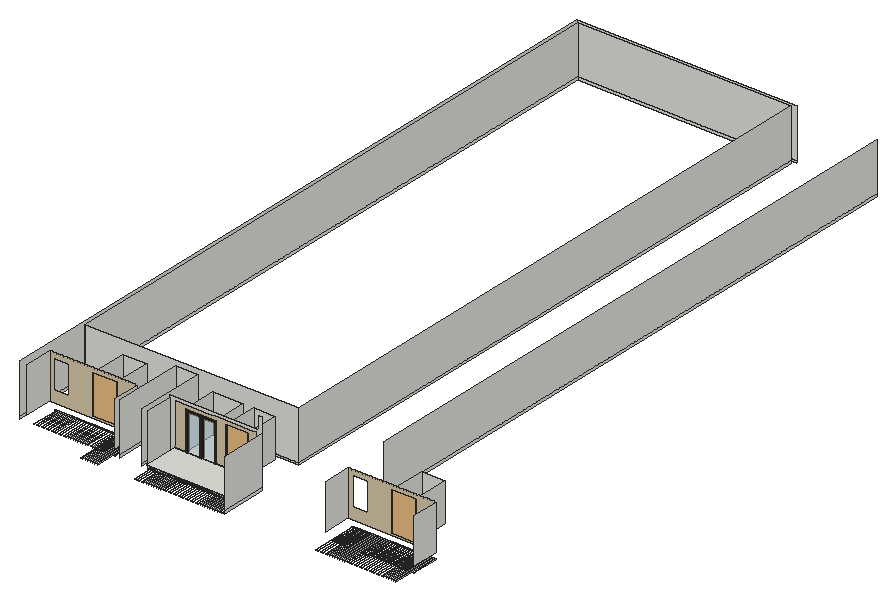
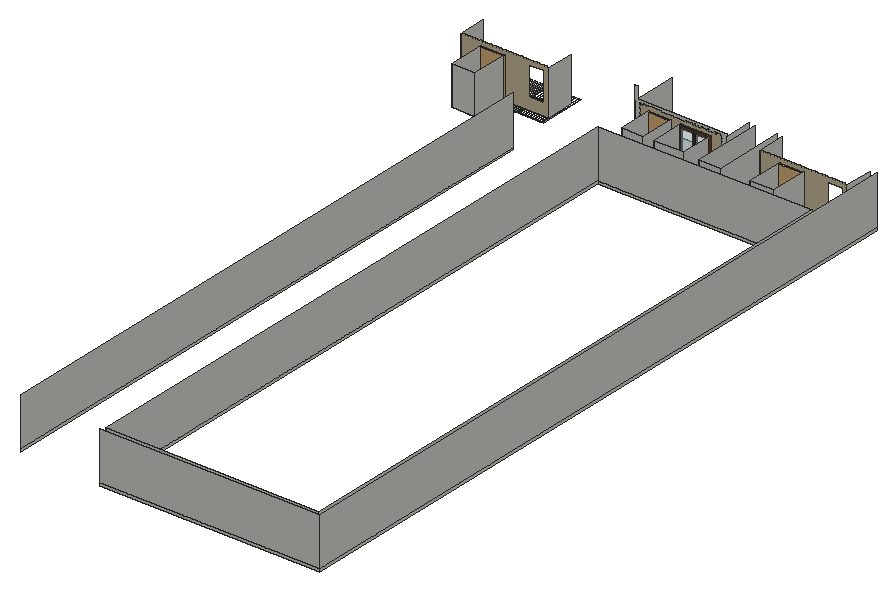
# SketchUp Ruby script. Lengths in inches.
U = 1.inch
M = Sketchup.active_model
def pt(a) = Geom::Point3d.new(a.map { |v| v * U })
def face(e, loops, mat)
  f = e.add_face(loops[0].map { |a| pt(a) })
  loops[1..].each { |l| e.add_face(l.map { |a| pt(a) }).erase! }
  f.material = f.back_material = mat if mat
  f
end
# faces: each face lists its corners as indices into pts; further lists are holes
def faces(e, pts, list, mat = nil) = list.each { |f| face(e, (f[0].is_a?(Array) ? f : [f]).map { |l| l.map { |i| pts[i] } }, mat) }
# xy, xz, yz: faces in a plane at the given z, y or x. An outline is a flat list of corners, or four numbers for a rectangle; further outlines are holes
def ring(l) = l.size == 4 ? [[l[0], l[1]], [l[2], l[1]], [l[2], l[3]], [l[0], l[3]]] : l.each_slice(2).to_a
def flat(e, list, mat, &to3) = list.each { |f| face(e, (f[0].is_a?(Array) ? f : [f]).map { |l| ring(l).map { |u, v| to3.(u, v) } }, mat) }
def xy(e, z, list, mat = nil) = flat(e, list, mat) { |x, y| [x, y, z] }
def xz(e, y, list, mat = nil) = flat(e, list, mat) { |x, z| [x, y, z] }
def yz(e, x, list, mat = nil) = flat(e, list, mat) { |y, z| [x, y, z] }
def lines(e, pts, list) = list.each { |a, b| e.add_line(pt(pts[a]), pt(pts[b])) }
# prism: a flat outline (further loops are holes) pulled along v
def prism(e, loops, v, mat = nil)
  f = face(e, loops, mat); d = Geom::Vector3d.new(v.map { |x| x * U })
  f.pushpull(f.normal.samedirection?(d) ? d.length : -d.length)
end
def box(e, o, s, mat = nil) = prism(e, [[o, [o[0] + s[0], o[1], o[2]], [o[0] + s[0], o[1] + s[1], o[2]], [o[0], o[1] + s[1], o[2]]]], [0, 0, s[2]], mat)
def at(x, y, z, deg = 0) = Geom::Transformation.translation(pt([x, y, z])) * Geom::Transformation.rotation(ORIGIN, Z_AXIS, deg.degrees)
def axes(o, x, y, z) = Geom::Transformation.new([*x, 0, *y, 0, *z, 0, *pt(o).to_a, 1])
def part(name) = M.definitions.add(name)
# library, detail: a bought-in or finely detailed component or shape, given as its bounding box
def library(name, o, s) = part(name).tap { |d| box(d.entities, o, s) }
def detail(e, o, s) = box(e.add_group.entities, o, s)
def put(e, d, t, mat = nil) = e.add_instance(d, t).tap { |i| i.material = mat if mat }
def group(e, t, mat = nil) = e.add_group.tap { |g| g.transformation = t; g.material = mat if mat }.entities
root = M.entities
M.materials.add("[Field Square Tile]").color = [216, 200, 168]
M.materials.add("[Translucent Glass Safety]").color = [204, 235, 244]
M.materials["[Translucent Glass Safety]"].alpha = 0.5
M.materials.add("[Wood Floor Parquet]").color = [140, 85, 37]
M.materials.add("[Wood Veneer 01]").color = [51, 28, 15]
M.materials.add("[Wood Veneer 01]1").color = [120, 70, 37]
c1 = library("元件\#5",[-4.39,0,0],[5.37,35.83,90.55])
c2 = part("Component\#1")
xy(c2.entities,0,[[0,0,6,48]],"[Wood Veneer 01]1")
xy(c2.entities,4,[[0,4,1.8125,44],[1.8125,4,6,44]])
xy(c2.entities,80,[[0,4,1.8125,44],[1.8125,4,6,44]])
xy(c2.entities,84,[[0,0,6,48]],"[Wood Veneer 01]1")
xz(c2.entities,0,[[0,0,6,84]],"[Wood Veneer 01]1")
xz(c2.entities,4,[[0,4,1.8125,80],[1.8125,4,6,80]])
xz(c2.entities,44,[[0,4,1.8125,80],[1.8125,4,6,80]])
xz(c2.entities,48,[[0,0,6,84]],"[Wood Veneer 01]1")
yz(c2.entities,0,[[[0,0,48,84],[4,4,44,80]]],"[Wood Veneer 01]1")
yz(c2.entities,1.8125,[[4,4,44,80]],"[Translucent Glass Safety]")
yz(c2.entities,6,[[[0,0,48,84],[4,4,44,80]]],"[Wood Veneer 01]")
c3 = part("Group\#3")
put(c3.entities,c2,at(0,0,0),"[Wood Veneer 01]")
g1 = group(c3.entities,at(0,48,0),"[Wood Veneer 01]")
xy(g1,0,[[0,0,6,48]],"[Wood Veneer 01]1")
xy(g1,4,[[0,4,1.8125,44],[1.8125,4,6,44]])
xy(g1,80,[[0,4,1.8125,44],[1.8125,4,6,44]])
xy(g1,84,[[0,0,6,48]],"[Wood Veneer 01]1")
xz(g1,0,[[0,0,6,84]],"[Wood Veneer 01]1")
xz(g1,4,[[0,4,1.8125,80],[1.8125,4,6,80]])
xz(g1,44,[[0,4,1.8125,80],[1.8125,4,6,80]])
xz(g1,48,[[0,0,6,84]],"[Wood Veneer 01]1")
yz(g1,0,[[[0,0,48,84],[4,4,44,80]]],"[Wood Veneer 01]1")
yz(g1,1.8125,[[4,4,44,80]],"[Translucent Glass Safety]")
yz(g1,6,[[[0,0,48,84],[4,4,44,80]]],"[Wood Veneer 01]")
xy(root,254.6875,[[614.76,246.64,616.96,361.27],[616.96,246.64,622,361.27]])
xy(root,274.4375,[[207.81,361.27,266.47,452.64],[941.37,361.27,1000.03,452.64]])
xy(root,275.125,[[409.32,273.33,609.07,361.27],[435.49,361.27,509.74,445.08],[534.92,361.27,587.67,445.08]])
xz(root,361.27,[[256.68,253.5625,261.43,254.6875],[262.68,253.5625,267.43,254.6875],[268.68,253.5625,273.43,254.6875],[274.68,253.5625,279.43,254.6875],[280.68,253.5625,285.43,254.6875],
  [286.68,253.5625,291.43,254.6875],[292.68,253.5625,297.43,254.6875],[298.68,253.5625,303.43,254.6875],[304.68,253.5625,309.43,254.6875],[310.68,253.5625,315.43,254.6875],
  [990.25,253.5625,995,254.6875],[996.25,253.5625,1001,254.6875],[1002.25,253.5625,1007,254.6875],[1008.25,253.5625,1013,254.6875],[1014.25,253.5625,1019,254.6875],
  [1020.25,253.5625,1025,254.6875],[1026.25,253.5625,1031,254.6875],[1032.25,253.5625,1037,254.6875],[1038.25,253.5625,1043,254.6875],[1044.25,253.5625,1049,254.6875],
  [244.68,253.875,249.43,254.625],[250.68,253.875,255.43,254.6875],[978.25,253.875,983,254.625],[984.25,253.875,989,254.6875],[112.68,253.9375,117.43,254.6875],
  [118.68,253.9375,123.43,254.6875],[124.68,253.9375,129.43,254.6875],[130.68,253.9375,135.43,254.6875],[136.68,253.9375,141.43,254.6875],[142.68,253.9375,147.43,254.6875],
  [148.68,253.9375,153.43,254.6875],[154.68,253.9375,159.43,254.6875],[160.68,253.9375,165.43,254.6875],[166.68,253.9375,171.43,254.6875],[172.68,253.9375,177.43,254.6875],
  [178.68,253.9375,183.43,254.6875],[184.68,253.9375,189.43,254.6875],[190.68,253.9375,195.43,254.6875],[196.68,253.9375,201.43,254.6875],[202.68,253.9375,207.43,254.6875],
  [208.68,253.9375,213.43,254.6875],[214.68,253.9375,219.43,254.6875],[220.68,253.9375,225.43,254.6875],[226.68,253.9375,231.43,254.6875],[232.68,253.9375,237.43,254.6875],
  [238.68,253.9375,243.43,254.6875],[396.57,253.9375,400.96,254.6875],[402.57,253.9375,406.96,254.6875],[408.57,253.9375,412.96,254.6875],[414.57,253.9375,418.96,254.6875],
  [420.57,253.9375,424.96,254.6875],[426.57,253.9375,430.96,254.6875],[432.57,253.9375,436.96,254.6875],[438.57,253.9375,442.96,254.6875],[444.57,253.9375,448.96,254.6875],
  [450.57,253.9375,454.96,254.6875],[456.57,253.9375,460.96,254.6875],[462.57,253.9375,466.96,254.6875],[468.57,253.9375,472.96,254.6875],[474.57,253.9375,478.96,254.6875],
  [480.57,253.9375,484.96,254.6875],[486.57,253.9375,490.96,254.6875],[492.57,253.9375,496.96,254.6875],[498.57,253.9375,502.96,254.6875],[504.57,253.9375,508.96,254.6875],
  [510.57,253.9375,514.96,254.6875],[516.57,253.9375,520.96,254.6875],[522.57,253.9375,526.96,254.6875],[528.57,253.9375,532.96,254.6875],[534.57,253.9375,538.96,254.6875],
  [540.57,253.9375,544.96,254.6875],[546.57,253.9375,550.96,254.6875],[552.57,253.9375,556.96,254.6875],[558.57,253.9375,562.96,254.6875],[564.57,253.9375,568.96,254.6875],
  [570.57,253.9375,574.96,254.6875],[576.57,253.9375,580.96,254.6875],[582.57,253.9375,586.96,254.6875],[588.57,253.9375,592.96,254.6875],[594.57,253.9375,598.96,254.6875],
  [600.57,253.9375,604.96,254.6875],[606.57,253.9375,610.96,254.6875],[612.57,253.9375,614.76,254.6875],[846.25,253.9375,851,254.6875],[852.25,253.9375,857,254.6875],
  [858.25,253.9375,863,254.6875],[864.25,253.9375,869,254.6875],[870.25,253.9375,875,254.6875],[876.25,253.9375,881,254.6875],[882.25,253.9375,887,254.6875],
  [888.25,253.9375,893,254.6875],[894.25,253.9375,899,254.6875],[900.25,253.9375,905,254.6875],[906.25,253.9375,911,254.6875],[912.25,253.9375,917,254.6875],
  [918.25,253.9375,923,254.6875],[924.25,253.9375,929,254.6875],[930.25,253.9375,935,254.6875],[936.25,253.9375,941,254.6875],[942.25,253.9375,947,254.6875],
  [948.25,253.9375,953,254.6875],[954.25,253.9375,959,254.6875],[960.25,253.9375,965,254.6875],[966.25,253.9375,971,254.6875],[972.25,253.9375,977,254.6875],
  [244.68,254.625,249.43,254.6875],[978.25,254.625,983,254.6875],[[396.57,254.6875,396.57,386.6875,614.76,386.6875,614.76,416.75,622,416.75,622,254.6875],[435.49,260.6875,509.74,260.6875,509.74,275.125,534.92,275.125,534.92,260.6875,587.67,260.6875,587.67,275.125,609.07,275.125,609.07,380.6875,605.74,380.6875,605.74,380.1875,601.32,380.1875,601.32,380.6875,599.74,380.6875,599.74,380.1875,595.32,380.1875,595.32,380.6875,593.74,380.6875,593.74,380.1875,589.32,380.1875,589.32,380.6875,587.74,380.6875,587.74,380.1875,583.32,380.1875,583.32,380.6875,581.74,380.6875,581.74,380.1875,577.32,380.1875,577.32,380.6875,575.74,380.6875,575.74,380.1875,571.32,380.1875,571.32,380.6875,569.74,380.6875,569.74,380.0625,565.32,380.0625,565.32,380.6875,563.74,380.6875,563.74,380.0625,559.32,380.0625,559.32,380.6875,557.74,380.6875,557.74,380.0625,553.32,380.0625,553.32,380.6875,551.74,380.6875,551.74,380.0625,547.32,380.0625,547.32,380.6875,545.74,380.6875,545.74,380.0625,541.32,380.0625,541.32,380.6875,539.74,380.6875,539.74,380.0625,535.32,380.0625,535.32,380.6875,533.74,380.6875,533.74,380.0625,529.32,380.0625,529.32,380.6875,527.74,380.6875,527.74,380.0625,523.32,380.0625,523.32,380.6875,521.74,380.6875,521.74,380.0625,517.32,380.0625,517.32,380.6875,515.74,380.6875,515.74,380.0625,511.32,380.0625,511.32,380.6875,509.74,380.6875,509.74,380.0625,505.32,380.0625,505.32,380.6875,503.74,380.6875,503.74,379.5625,499.32,379.5625,499.32,380.6875,497.74,380.6875,497.74,379.5625,493.32,379.5625,493.32,380.6875,491.74,380.6875,491.74,379.5625,487.32,379.5625,487.32,380.6875,485.74,380.6875,485.74,379.5625,481.32,379.5625,481.32,380.6875,479.74,380.6875,479.74,379.5625,475.32,379.5625,475.32,380.6875,473.74,380.6875,473.74,379.5625,469.32,379.5625,469.32,380.6875,467.74,380.6875,467.74,379.5625,463.32,379.5625,463.32,380.6875,461.74,380.6875,461.74,379.5625,457.32,379.5625,457.32,380.6875,455.74,380.6875,455.74,379.5625,451.32,379.5625,451.32,380.6875,449.74,380.6875,449.74,379.5625,445.32,379.5625,445.32,380.6875,443.74,380.6875,443.74,379.5625,439.32,379.5625,439.32,380.6875,437.74,380.6875,437.74,379.5625,433.32,379.5625,433.32,380.6875,431.74,380.6875,431.74,379.5625,427.32,379.5625,427.32,380.6875,425.74,380.6875,425.74,379.5625,421.32,379.5625,421.32,380.6875,419.74,380.6875,419.74,379.5625,415.32,379.5625,415.32,380.6875,413.74,380.6875,413.74,379.5625,409.32,379.5625,409.32,275.125,435.49,275.125]],[435.49,260.6875,509.74,275.125],[534.92,260.6875,587.67,275.125]])
xz(root,361.27,[[[100.18,269.0625,315.43,269.0625,315.43,378.875,310.4,378.875,310.4,380.6875,307.02,380.6875,307.02,378.875,301.98,378.875,301.98,380.6875,298.61,380.6875,298.61,378.875,293.57,378.875,293.57,380.6875,290.2,380.6875,290.2,378.875,285.16,378.875,285.16,380.6875,281.78,380.6875,281.78,378.875,276.75,378.875,276.75,380.6875,273.37,380.6875,273.37,378.875,268.33,378.875,268.33,380.6875,264.96,380.6875,264.96,378.875,259.92,378.875,259.92,380.6875,256.55,380.6875,256.55,378.875,251.51,378.875,251.51,380.6875,248.13,380.6875,248.13,378.875,243.1,378.875,243.1,380.6875,239.72,380.6875,239.72,378.875,234.68,378.875,234.68,380.6875,231.31,380.6875,231.31,378.875,226.27,378.875,226.27,380.6875,222.89,380.6875,222.89,378.875,217.86,378.875,217.86,380.6875,214.48,380.6875,214.48,378.875,209.44,378.875,209.44,380.6875,206.07,380.6875,206.07,378.875,201.03,378.875,201.03,380.6875,197.66,380.6875,197.66,378.875,192.62,378.875,192.62,380.6875,189.24,380.6875,189.24,378.875,184.21,378.875,184.21,380.6875,180.83,380.6875,180.83,378.875,175.79,378.875,175.79,380.6875,172.42,380.6875,172.42,378.875,167.38,378.875,167.38,380.6875,164.01,380.6875,164.01,378.875,158.97,378.875,158.97,380.6875,155.59,380.6875,155.59,378.875,150.55,378.875,150.55,380.6875,147.18,380.6875,147.18,378.875,142.14,378.875,142.14,380.6875,138.77,380.6875,138.77,378.875,133.73,378.875,133.73,380.6875,130.35,380.6875,130.35,378.875,125.32,378.875,125.32,380.6875,121.94,380.6875,121.94,378.875,116.9,378.875,116.9,380.6875,113.53,380.6875,113.53,378.875,108.49,378.875,108.49,380.6875,105.12,380.6875,105.12,378.875,100.18,378.875],[207.81,274.4375,266.47,369.36],[111.92,297.24,149.24,369.37]],[[833.74,269.0625,1049,269.0625,1049,378.875,1043.96,378.875,1043.96,380.6875,1040.58,380.6875,1040.58,378.875,1035.55,378.875,1035.55,380.6875,1032.17,380.6875,1032.17,378.875,1027.13,378.875,1027.13,380.6875,1023.76,380.6875,1023.76,378.875,1018.72,378.875,1018.72,380.6875,1015.35,380.6875,1015.35,378.875,1010.31,378.875,1010.31,380.6875,1006.93,380.6875,1006.93,378.875,1001.9,378.875,1001.9,380.6875,998.52,380.6875,998.52,378.875,993.48,378.875,993.48,380.6875,990.11,380.6875,990.11,378.875,985.07,378.875,985.07,380.6875,981.7,380.6875,981.7,378.875,976.66,378.875,976.66,380.6875,973.28,380.6875,973.28,378.875,968.24,378.875,968.24,380.6875,964.87,380.6875,964.87,378.875,959.83,378.875,959.83,380.6875,956.46,380.6875,956.46,378.875,951.42,378.875,951.42,380.6875,948.04,380.6875,948.04,378.875,943.01,378.875,943.01,380.6875,939.63,380.6875,939.63,378.875,934.59,378.875,934.59,380.6875,931.22,380.6875,931.22,378.875,926.18,378.875,926.18,380.6875,922.81,380.6875,922.81,378.875,917.77,378.875,917.77,380.6875,914.39,380.6875,914.39,378.875,909.36,378.875,909.36,380.6875,905.98,380.6875,905.98,378.875,900.94,378.875,900.94,380.6875,897.57,380.6875,897.57,378.875,892.53,378.875,892.53,380.6875,889.16,380.6875,889.16,378.875,884.12,378.875,884.12,380.6875,880.74,380.6875,880.74,378.875,875.7,378.875,875.7,380.6875,872.33,380.6875,872.33,378.875,867.29,378.875,867.29,380.6875,863.92,380.6875,863.92,378.875,858.88,378.875,858.88,380.6875,855.5,380.6875,855.5,378.875,850.47,378.875,850.47,380.6875,847.09,380.6875,847.09,378.875,842.05,378.875,842.05,380.6875,838.68,380.6875,838.68,378.875,833.74,378.875],[941.37,274.4375,1000.03,369.36],[845.49,297.24,882.8,369.37]],[409.32,275.125,435.49,275.125,435.49,369.625,509.74,369.625,509.74,275.125,534.92,275.125,534.92,369.6875,587.67,369.6875,587.67,275.125,609.07,275.125,609.07,380.6875,605.74,380.6875,605.74,380.1875,601.32,380.1875,601.32,380.6875,599.74,380.6875,599.74,380.1875,595.32,380.1875,595.32,380.6875,593.74,380.6875,593.74,380.1875,589.32,380.1875,589.32,380.6875,587.74,380.6875,587.74,380.1875,583.32,380.1875,583.32,380.6875,581.74,380.6875,581.74,380.1875,577.32,380.1875,577.32,380.6875,575.74,380.6875,575.74,380.1875,571.32,380.1875,571.32,380.6875,569.74,380.6875,569.74,380.0625,565.32,380.0625,565.32,380.6875,563.74,380.6875,563.74,380.0625,559.32,380.0625,559.32,380.6875,557.74,380.6875,557.74,380.0625,553.32,380.0625,553.32,380.6875,551.74,380.6875,551.74,380.0625,547.32,380.0625,547.32,380.6875,545.74,380.6875,545.74,380.0625,541.32,380.0625,541.32,380.6875,539.74,380.6875,539.74,380.0625,535.32,380.0625,535.32,380.6875,533.74,380.6875,533.74,380.0625,529.32,380.0625,529.32,380.6875,527.74,380.6875,527.74,380.0625,523.32,380.0625,523.32,380.6875,521.74,380.6875,521.74,380.0625,517.32,380.0625,517.32,380.6875,515.74,380.6875,515.74,380.0625,511.32,380.0625,511.32,380.6875,509.74,380.6875,509.74,380.0625,505.32,380.0625,505.32,380.6875,503.74,380.6875,503.74,379.5625,499.32,379.5625,499.32,380.6875,497.74,380.6875,497.74,379.5625,493.32,379.5625,493.32,380.6875,491.74,380.6875,491.74,379.5625,487.32,379.5625,487.32,380.6875,485.74,380.6875,485.74,379.5625,481.32,379.5625,481.32,380.6875,479.74,380.6875,479.74,379.5625,475.32,379.5625,475.32,380.6875,473.74,380.6875,473.74,379.5625,469.32,379.5625,469.32,380.6875,467.74,380.6875,467.74,379.5625,463.32,379.5625,463.32,380.6875,461.74,380.6875,461.74,379.5625,457.32,379.5625,457.32,380.6875,455.74,380.6875,455.74,379.5625,451.32,379.5625,451.32,380.6875,449.74,380.6875,449.74,379.5625,445.32,379.5625,445.32,380.6875,443.74,380.6875,443.74,379.5625,439.32,379.5625,439.32,380.6875,437.74,380.6875,437.74,379.5625,433.32,379.5625,433.32,380.6875,431.74,380.6875,431.74,379.5625,427.32,379.5625,427.32,380.6875,425.74,380.6875,425.74,379.5625,421.32,379.5625,421.32,380.6875,419.74,380.6875,419.74,379.5625,415.32,379.5625,415.32,380.6875,413.74,380.6875,413.74,379.5625,409.32,379.5625]],"[Field Square Tile]")
xz(root,445.08,[[435.49,275.125,509.74,369.625],[534.92,275.125,587.67,369.6875]])
xz(root,452.64,[[207.81,274.4375,266.47,369.36],[941.37,274.4375,1000.03,369.36]])
xz(root,465.02,[[328.03,254.6875,382.74,260.6875],[328.03,260.6875,382.74,380.6875]])
xz(root,483.79,[[90.36,254.6875,614.76,260.6875],[90.36,260.6875,614.76,380.6875]])
xz(root,1996.66,[[90.36,254.6875,614.76,260.6875],[90.36,260.6875,614.76,380.6875]])
xz(root,2003.89,[[83.125,254.6875,622,260.6875],[83.125,260.6875,622,380.6875]])
yz(root,83.125,[[293.46,254.6875,2003.89,260.6875],[293.46,260.6875,2003.89,380.6875]])
yz(root,90.36,[[483.79,254.6875,1996.66,260.6875],[483.79,260.6875,1996.66,380.6875]])
yz(root,100.18,[[293.46,269.0625,361.27,378.875]])
yz(root,117.43,[[293.45,253.9375,361.27,254.6875]])
yz(root,123.43,[[293.45,253.9375,361.27,254.6875]])
yz(root,129.43,[[293.45,253.9375,361.27,254.6875]])
yz(root,135.43,[[293.45,253.9375,361.27,254.6875]])
yz(root,141.43,[[293.45,253.9375,361.27,254.6875]])
yz(root,147.43,[[293.45,253.9375,361.27,254.6875]])
yz(root,153.43,[[293.45,253.9375,361.27,254.6875]])
yz(root,159.43,[[293.45,253.9375,361.27,254.6875]])
yz(root,165.43,[[293.45,253.9375,361.27,254.6875]])
yz(root,171.43,[[293.45,253.9375,361.27,254.6875]])
yz(root,177.43,[[293.45,253.9375,361.27,254.6875]])
yz(root,183.43,[[293.45,253.9375,361.27,254.6875]])
yz(root,189.43,[[293.45,253.9375,361.27,254.6875]])
yz(root,195.43,[[293.45,253.9375,361.27,254.6875]])
yz(root,201.43,[[293.45,253.9375,361.27,254.6875]])
yz(root,207.43,[[293.45,253.9375,361.27,254.6875]])
yz(root,207.81,[[361.27,274.4375,452.64,369.36]])
yz(root,213.43,[[293.45,253.9375,361.27,254.6875]])
yz(root,219.43,[[293.45,253.9375,361.27,254.6875]])
yz(root,225.43,[[293.45,253.9375,361.27,254.6875]])
yz(root,231.43,[[293.45,253.9375,361.27,254.6875]])
yz(root,237.43,[[293.45,253.9375,361.27,254.6875]])
yz(root,243.43,[[293.45,253.9375,361.27,254.6875]])
yz(root,249.43,[[293.45,253.875,361.27,254.625],[293.45,254.625,361.27,254.6875]])
yz(root,255.43,[[293.45,253.875,361.27,254.6875]])
yz(root,261.43,[[293.45,253.5625,361.27,254.6875]])
yz(root,266.47,[[361.27,274.4375,452.64,369.36]])
yz(root,267.43,[[293.45,253.5625,361.27,254.6875]])
yz(root,268.68,[[246.64,253.5625,361.27,254.6875]])
yz(root,273.43,[[293.45,253.5625,361.27,254.6875]])
yz(root,274.68,[[246.64,253.5625,361.27,254.6875]])
yz(root,279.43,[[293.45,253.5625,361.27,254.6875]])
yz(root,280.68,[[246.64,253.5625,361.27,254.6875]])
yz(root,285.43,[[293.45,253.5625,361.27,254.6875]])
yz(root,286.68,[[246.64,253.5625,361.27,254.6875]])
yz(root,291.43,[[293.45,253.5625,361.27,254.6875]])
yz(root,292.68,[[246.64,253.5625,361.27,254.6875]])
yz(root,297.43,[[293.45,253.5625,361.27,254.6875]])
yz(root,298.68,[[246.64,253.5625,361.27,254.6875]])
yz(root,303.43,[[293.45,253.5625,361.27,254.6875]])
yz(root,304.68,[[246.64,253.5625,361.27,254.6875]])
yz(root,309.43,[[293.45,253.5625,361.27,254.6875]])
yz(root,310.68,[[246.64,253.5625,361.27,254.6875]])
yz(root,315.43,[[293.45,253.5625,361.27,254.6875],[293.45,269.0625,361.27,378.875]])
yz(root,328.03,[[293.45,254.6875,465.02,260.6875],[293.45,260.6875,465.02,380.6875]])
yz(root,382.74,[[293.45,254.6875,465.02,260.6875],[293.45,260.6875,465.02,380.6875]])
yz(root,396.57,[[293.45,253.9375,361.27,254.6875],[293.45,254.6875,361.27,260.6875],[293.45,260.6875,361.27,380.6875]])
yz(root,400.96,[[246.64,253.9375,361.27,254.6875]])
yz(root,402.57,[[293.45,253.9375,361.27,254.6875]])
yz(root,406.96,[[246.64,253.9375,361.27,254.6875]])
yz(root,408.57,[[293.45,253.9375,361.27,254.6875]])
yz(root,412.96,[[246.64,253.9375,361.27,254.6875]])
yz(root,414.57,[[293.45,253.9375,361.27,254.6875]])
yz(root,418.96,[[246.64,253.9375,361.27,254.6875]])
yz(root,420.57,[[293.45,253.9375,361.27,254.6875]])
yz(root,424.96,[[246.64,253.9375,361.27,254.6875]])
yz(root,426.57,[[293.45,253.9375,361.27,254.6875]])
yz(root,430.96,[[246.64,253.9375,361.27,254.6875]])
yz(root,432.57,[[293.45,253.9375,361.27,254.6875]])
yz(root,435.49,[[361.27,275.125,445.08,369.625]])
yz(root,436.96,[[246.64,253.9375,361.27,254.6875]])
yz(root,438.57,[[293.45,253.9375,361.27,254.6875]])
yz(root,442.96,[[246.64,253.9375,361.27,254.6875]])
yz(root,444.57,[[293.45,253.9375,361.27,254.6875]])
yz(root,448.96,[[246.64,253.9375,361.27,254.6875]])
yz(root,450.57,[[293.45,253.9375,361.27,254.6875]])
yz(root,454.96,[[246.64,253.9375,361.27,254.6875]])
yz(root,456.57,[[293.45,253.9375,361.27,254.6875]])
yz(root,460.96,[[246.64,253.9375,361.27,254.6875]])
yz(root,462.57,[[293.45,253.9375,361.27,254.6875]])
yz(root,466.96,[[246.64,253.9375,361.27,254.6875]])
yz(root,468.57,[[293.45,253.9375,361.27,254.6875]])
yz(root,472.96,[[246.64,253.9375,361.27,254.6875]])
yz(root,474.57,[[293.45,253.9375,361.27,254.6875]])
yz(root,478.96,[[246.64,253.9375,361.27,254.6875]])
yz(root,480.57,[[293.45,253.9375,361.27,254.6875]])
yz(root,484.96,[[246.64,253.9375,361.27,254.6875]])
yz(root,486.57,[[293.45,253.9375,361.27,254.6875]])
yz(root,490.96,[[246.64,253.9375,361.27,254.6875]])
yz(root,492.57,[[293.45,253.9375,361.27,254.6875]])
yz(root,496.96,[[246.64,253.9375,361.27,254.6875]])
yz(root,498.57,[[293.45,253.9375,361.27,254.6875]])
yz(root,502.96,[[246.64,253.9375,361.27,254.6875]])
yz(root,504.57,[[293.45,253.9375,361.27,254.6875]])
yz(root,508.96,[[246.64,253.9375,361.27,254.6875]])
yz(root,509.74,[[361.27,275.125,445.08,369.625]])
yz(root,510.57,[[293.45,253.9375,361.27,254.6875]])
yz(root,514.96,[[246.64,253.9375,361.27,254.6875]])
yz(root,516.57,[[293.45,253.9375,361.27,254.6875]])
yz(root,520.96,[[246.64,253.9375,361.27,254.6875]])
yz(root,522.57,[[293.45,253.9375,361.27,254.6875]])
yz(root,526.96,[[246.64,253.9375,361.27,254.6875]])
yz(root,528.57,[[293.45,253.9375,361.27,254.6875]])
yz(root,532.96,[[246.64,253.9375,361.27,254.6875]])
yz(root,534.57,[[293.45,253.9375,361.27,254.6875]])
yz(root,534.92,[[361.27,275.125,445.08,369.6875]])
yz(root,538.96,[[246.64,253.9375,361.27,254.6875]])
yz(root,540.57,[[293.45,253.9375,361.27,254.6875]])
yz(root,544.96,[[246.64,253.9375,361.27,254.6875]])
yz(root,546.57,[[293.45,253.9375,361.27,254.6875]])
yz(root,550.96,[[246.64,253.9375,361.27,254.6875]])
yz(root,552.57,[[293.45,253.9375,361.27,254.6875]])
yz(root,556.96,[[246.64,253.9375,361.27,254.6875]])
yz(root,558.57,[[293.45,253.9375,361.27,254.6875]])
yz(root,562.96,[[246.64,253.9375,361.27,254.6875]])
yz(root,564.57,[[293.45,253.9375,361.27,254.6875]])
yz(root,568.96,[[246.64,253.9375,361.27,254.6875]])
yz(root,570.57,[[293.45,253.9375,361.27,254.6875]])
yz(root,574.96,[[246.64,253.9375,361.27,254.6875]])
yz(root,576.57,[[293.45,253.9375,361.27,254.6875]])
yz(root,580.96,[[246.64,253.9375,361.27,254.6875]])
yz(root,582.57,[[293.45,253.9375,361.27,254.6875]])
yz(root,586.96,[[246.64,253.9375,361.27,254.6875]])
yz(root,587.67,[[361.27,275.125,445.08,369.6875]])
yz(root,588.57,[[293.45,253.9375,361.27,254.6875]])
yz(root,592.96,[[246.64,253.9375,361.27,254.6875]])
yz(root,594.57,[[293.45,253.9375,361.27,254.6875]])
yz(root,598.96,[[246.64,253.9375,361.27,254.6875]])
yz(root,600.57,[[293.45,253.9375,361.27,254.6875]])
yz(root,604.96,[[246.64,253.9375,361.27,254.6875]])
yz(root,606.57,[[293.45,253.9375,361.27,254.6875]])
yz(root,610.96,[[246.64,253.9375,361.27,254.6875]])
yz(root,612.57,[[293.45,253.9375,361.27,254.6875]])
yz(root,614.76,[[246.64,253.9375,361.27,254.6875],[483.79,254.6875,1996.66,260.6875],[483.79,260.6875,1996.66,380.6875]])
yz(root,622,[[246.64,254.6875,361.27,260.6875],[246.64,260.6875,361.27,380.6875]])
yz(root,823.93,[[483.79,254.6875,1996.66,260.6875],[483.79,260.6875,1996.66,380.6875]])
yz(root,833.74,[[293.46,269.0625,361.27,378.875]])
yz(root,846.25,[[246.64,253.9375,361.27,254.6875]])
yz(root,851,[[293.45,253.9375,361.27,254.6875]])
yz(root,852.25,[[246.64,253.9375,361.27,254.6875]])
yz(root,857,[[293.45,253.9375,361.27,254.6875]])
yz(root,858.25,[[246.64,253.9375,361.27,254.6875]])
yz(root,863,[[293.45,253.9375,361.27,254.6875]])
yz(root,864.25,[[246.64,253.9375,361.27,254.6875]])
yz(root,869,[[293.45,253.9375,361.27,254.6875]])
yz(root,870.25,[[246.64,253.9375,361.27,254.6875]])
yz(root,875,[[293.45,253.9375,361.27,254.6875]])
yz(root,876.25,[[246.64,253.9375,361.27,254.6875]])
yz(root,881,[[293.45,253.9375,361.27,254.6875]])
yz(root,882.25,[[246.64,253.9375,361.27,254.6875]])
yz(root,887,[[293.45,253.9375,361.27,254.6875]])
yz(root,888.25,[[246.64,253.9375,361.27,254.6875]])
yz(root,893,[[293.45,253.9375,361.27,254.6875]])
yz(root,894.25,[[246.64,253.9375,361.27,254.6875]])
yz(root,899,[[293.45,253.9375,361.27,254.6875]])
yz(root,900.25,[[246.64,253.9375,361.27,254.6875]])
yz(root,905,[[293.45,253.9375,361.27,254.6875]])
yz(root,906.25,[[246.64,253.9375,361.27,254.6875]])
yz(root,911,[[293.45,253.9375,361.27,254.6875]])
yz(root,912.25,[[246.64,253.9375,361.27,254.6875]])
yz(root,917,[[293.45,253.9375,361.27,254.6875]])
yz(root,918.25,[[246.64,253.9375,361.27,254.6875]])
yz(root,923,[[293.45,253.9375,361.27,254.6875]])
yz(root,924.25,[[246.64,253.9375,361.27,254.6875]])
yz(root,929,[[293.45,253.9375,361.27,254.6875]])
yz(root,930.25,[[246.64,253.9375,361.27,254.6875]])
yz(root,935,[[293.45,253.9375,361.27,254.6875]])
yz(root,936.25,[[246.64,253.9375,361.27,254.6875]])
yz(root,941,[[293.45,253.9375,361.27,254.6875]])
yz(root,941.37,[[361.27,274.4375,452.64,369.36]])
yz(root,942.25,[[246.64,253.9375,361.27,254.6875]])
yz(root,947,[[293.45,253.9375,361.27,254.6875]])
yz(root,948.25,[[246.64,253.9375,361.27,254.6875]])
yz(root,953,[[293.45,253.9375,361.27,254.6875]])
yz(root,954.25,[[246.64,253.9375,361.27,254.6875]])
yz(root,959,[[293.45,253.9375,361.27,254.6875]])
yz(root,960.25,[[246.64,253.9375,361.27,254.6875]])
yz(root,965,[[293.45,253.9375,361.27,254.6875]])
yz(root,966.25,[[246.64,253.9375,361.27,254.6875]])
yz(root,971,[[293.45,253.9375,361.27,254.6875]])
yz(root,972.25,[[246.64,253.9375,361.27,254.6875]])
yz(root,977,[[293.45,253.9375,361.27,254.6875]])
yz(root,978.25,[[246.64,253.875,361.27,254.625],[246.64,254.625,361.27,254.6875]])
yz(root,983,[[293.45,253.875,361.27,254.625],[293.45,254.625,361.27,254.6875]])
yz(root,984.25,[[246.64,253.875,361.27,254.6875]])
yz(root,989,[[293.45,253.875,361.27,254.6875]])
yz(root,990.25,[[246.64,253.5625,361.27,254.6875]])
yz(root,995,[[293.45,253.5625,361.27,254.6875]])
yz(root,996.25,[[246.64,253.5625,361.27,254.6875]])
yz(root,1000.03,[[361.27,274.4375,452.64,369.36]])
yz(root,1001,[[293.45,253.5625,361.27,254.6875]])
yz(root,1002.25,[[246.64,253.5625,361.27,254.6875]])
yz(root,1007,[[293.45,253.5625,361.27,254.6875]])
yz(root,1008.25,[[246.64,253.5625,361.27,254.6875]])
yz(root,1013,[[293.45,253.5625,361.27,254.6875]])
yz(root,1014.25,[[246.64,253.5625,361.27,254.6875]])
yz(root,1019,[[293.45,253.5625,361.27,254.6875]])
yz(root,1020.25,[[246.64,253.5625,361.27,254.6875]])
yz(root,1025,[[293.45,253.5625,361.27,254.6875]])
yz(root,1026.25,[[246.64,253.5625,361.27,254.6875]])
yz(root,1031,[[293.45,253.5625,361.27,254.6875]])
yz(root,1032.25,[[246.64,253.5625,361.27,254.6875]])
yz(root,1037,[[293.45,253.5625,361.27,254.6875]])
yz(root,1038.25,[[246.64,253.5625,361.27,254.6875]])
yz(root,1043,[[293.45,253.5625,361.27,254.6875]])
yz(root,1044.25,[[246.64,253.5625,361.27,254.6875]])
yz(root,1049,[[293.45,253.5625,361.27,254.6875],[293.45,269.0625,361.27,378.875]])
put(root,c1,axes([207.81,361.64,274.4375],[0,-1,0],[1.63746,0,0],[0,0,1.04827]))
put(root,c1,axes([941.37,361.64,274.4375],[0,-1,0],[1.63746,0,0],[0,0,1.04827]))
put(root,c1,axes([535.46,362.12,260.6875],[0,-0.89,0],[1.45734,0,0],[0,0,1.20374]),"[Wood Floor Parquet]")
put(root,c3,axes([435.49,367.27,260.6875],[0,-1,0],[0.77344,0,0],[0,0,1.29687]))
